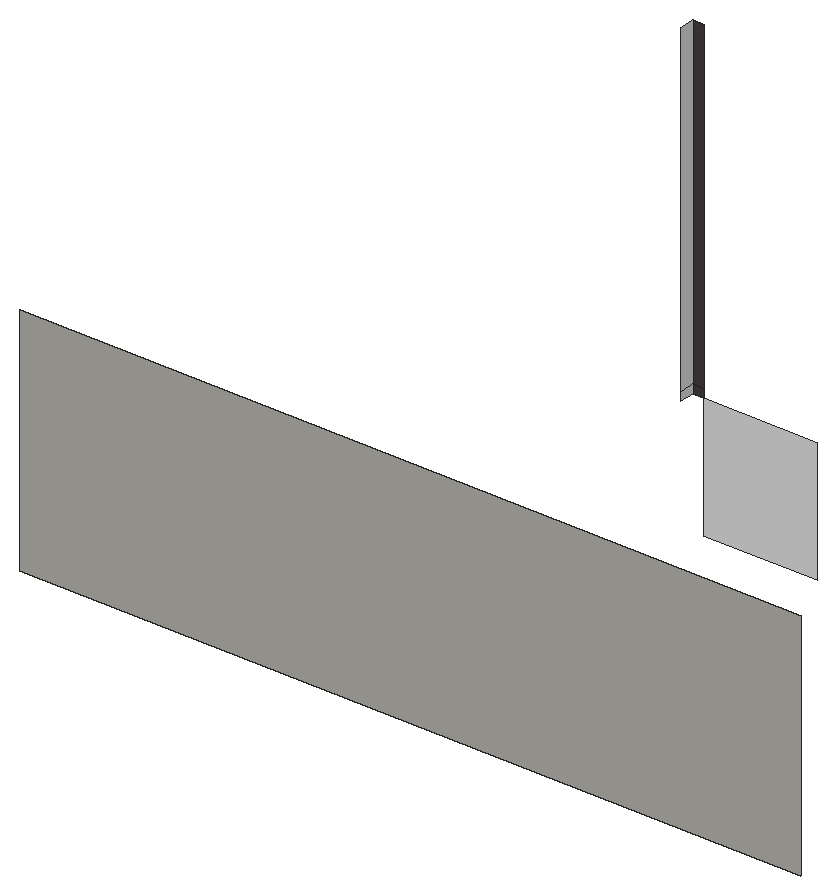
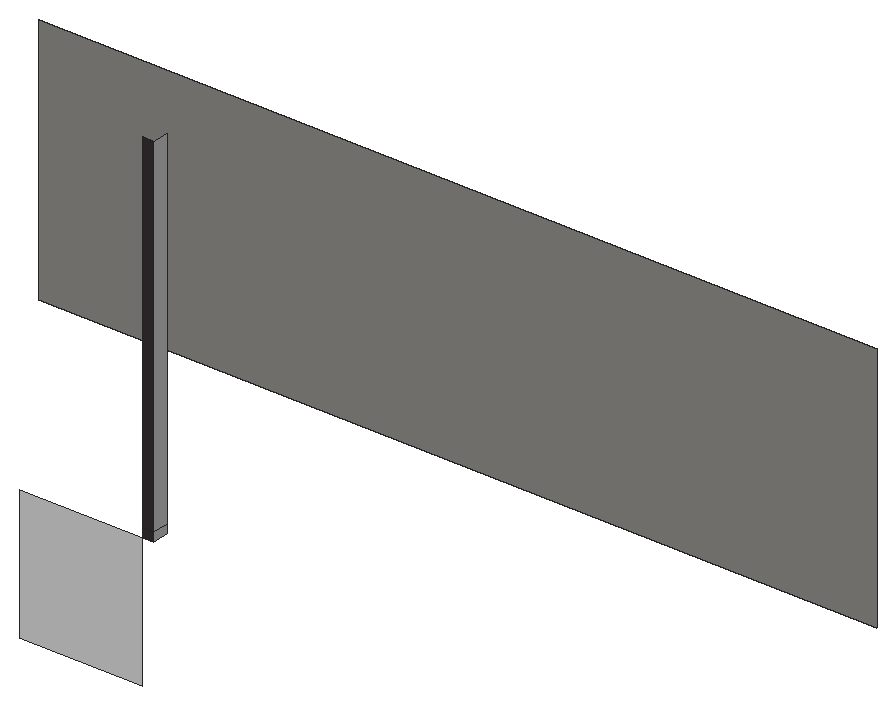
# SketchUp Ruby script. Lengths in inches.
U = 1.inch
M = Sketchup.active_model
def pt(a) = Geom::Point3d.new(a.map { |v| v * U })
def face(e, loops, mat)
  f = e.add_face(loops[0].map { |a| pt(a) })
  loops[1..].each { |l| e.add_face(l.map { |a| pt(a) }).erase! }
  f.material = f.back_material = mat if mat
  f
end
# faces: each face lists its corners as indices into pts; further lists are holes
def faces(e, pts, list, mat = nil) = list.each { |f| face(e, (f[0].is_a?(Array) ? f : [f]).map { |l| l.map { |i| pts[i] } }, mat) }
# xy, xz, yz: faces in a plane at the given z, y or x. An outline is a flat list of corners, or four numbers for a rectangle; further outlines are holes
def ring(l) = l.size == 4 ? [[l[0], l[1]], [l[2], l[1]], [l[2], l[3]], [l[0], l[3]]] : l.each_slice(2).to_a
def flat(e, list, mat, &to3) = list.each { |f| face(e, (f[0].is_a?(Array) ? f : [f]).map { |l| ring(l).map { |u, v| to3.(u, v) } }, mat) }
def xy(e, z, list, mat = nil) = flat(e, list, mat) { |x, y| [x, y, z] }
def xz(e, y, list, mat = nil) = flat(e, list, mat) { |x, z| [x, y, z] }
def yz(e, x, list, mat = nil) = flat(e, list, mat) { |y, z| [x, y, z] }
def lines(e, pts, list) = list.each { |a, b| e.add_line(pt(pts[a]), pt(pts[b])) }
# prism: a flat outline (further loops are holes) pulled along v
def prism(e, loops, v, mat = nil)
  f = face(e, loops, mat); d = Geom::Vector3d.new(v.map { |x| x * U })
  f.pushpull(f.normal.samedirection?(d) ? d.length : -d.length)
end
def box(e, o, s, mat = nil) = prism(e, [[o, [o[0] + s[0], o[1], o[2]], [o[0] + s[0], o[1] + s[1], o[2]], [o[0], o[1] + s[1], o[2]]]], [0, 0, s[2]], mat)
def at(x, y, z, deg = 0) = Geom::Transformation.translation(pt([x, y, z])) * Geom::Transformation.rotation(ORIGIN, Z_AXIS, deg.degrees)
def axes(o, x, y, z) = Geom::Transformation.new([*x, 0, *y, 0, *z, 0, *pt(o).to_a, 1])
def part(name) = M.definitions.add(name)
# library, detail: a bought-in or finely detailed component or shape, given as its bounding box
def library(name, o, s) = part(name).tap { |d| box(d.entities, o, s) }
def detail(e, o, s) = box(e.add_group.entities, o, s)
def put(e, d, t, mat = nil) = e.add_instance(d, t).tap { |i| i.material = mat if mat }
def group(e, t, mat = nil) = e.add_group.tap { |g| g.transformation = t; g.material = mat if mat }.entities
root = M.entities
M.materials.add("[Asphalt New]").color = [67, 60, 62]
M.materials.add("[Polished Concrete New]").color = [200, 200, 203]
M.materials.add("[Tile Travertine 2 inch]").color = [181, 178, 172]
M.materials.add("[Translucent Glass Gray]").color = [128, 128, 128]
M.materials["[Translucent Glass Gray]"].alpha = 0.5
xz(root,153.99,[[20.0625,7.8125,321.78,97.93]],"[Tile Travertine 2 inch]")
xz(root,304.24,[[160.07,52.25,164.29,55.45],[160.07,55.45,164.29,181.51]],"[Asphalt New]")
xz(root,304.24,[[164.29,4.22,208.29,52.25]],"[Translucent Glass Gray]")
yz(root,160.07,[[298.43,52.25,304.24,55.45],[298.43,55.45,304.24,181.51]],"[Polished Concrete New]")
